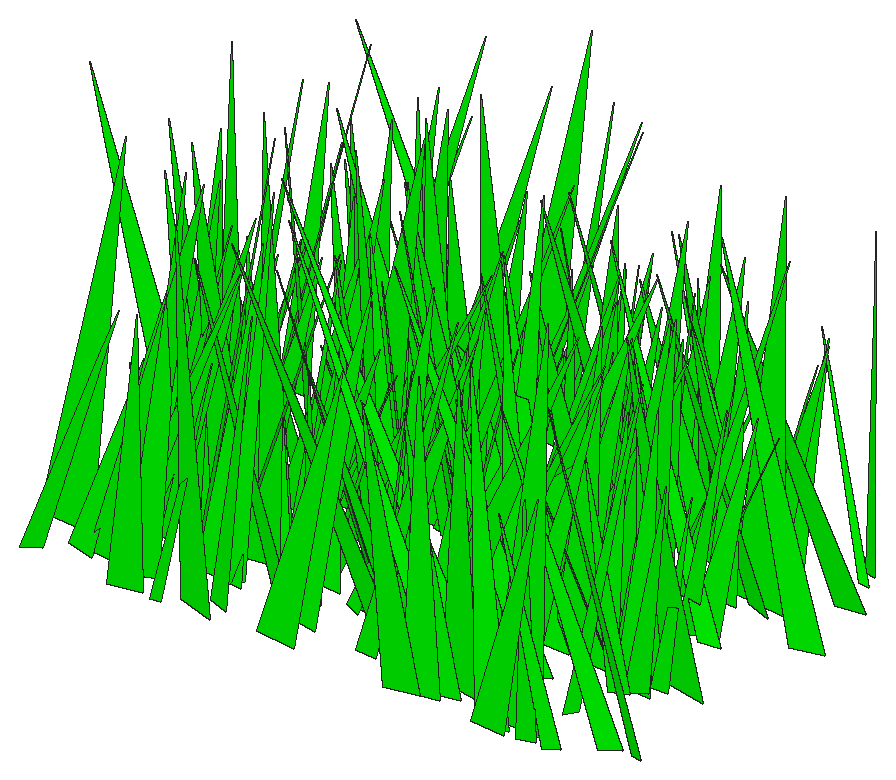
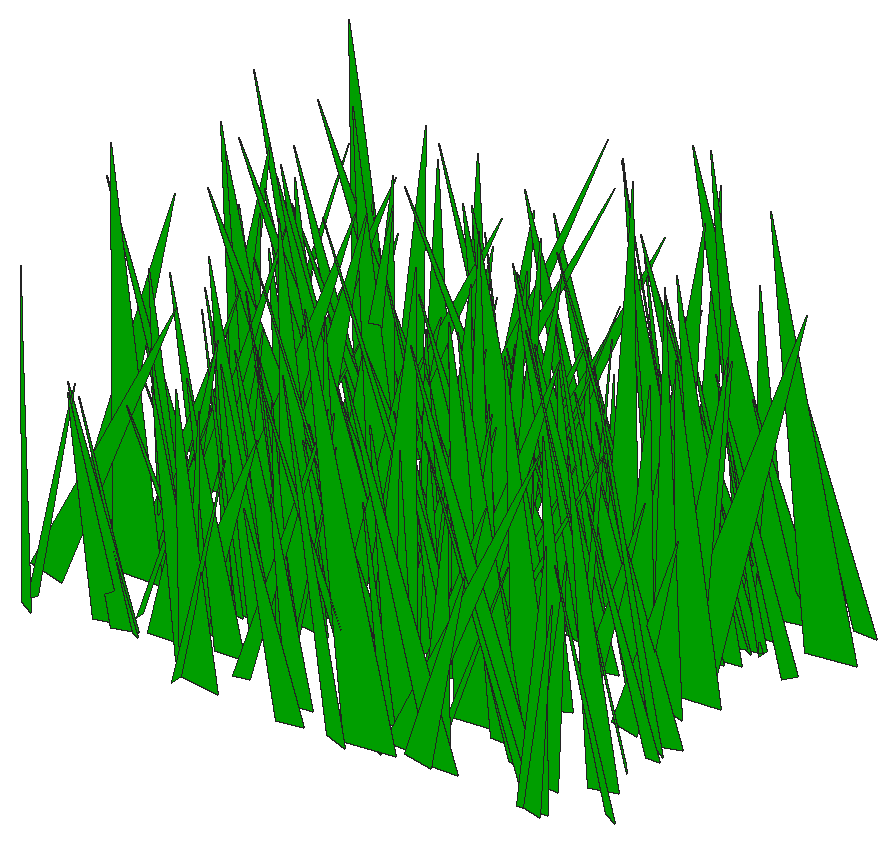
# SketchUp Ruby script. Lengths in inches.
U = 1.inch
M = Sketchup.active_model
def pt(a) = Geom::Point3d.new(a.map { |v| v * U })
def face(e, loops, mat)
  f = e.add_face(loops[0].map { |a| pt(a) })
  loops[1..].each { |l| e.add_face(l.map { |a| pt(a) }).erase! }
  f.material = f.back_material = mat if mat
  f
end
# faces: each face lists its corners as indices into pts; further lists are holes
def faces(e, pts, list, mat = nil) = list.each { |f| face(e, (f[0].is_a?(Array) ? f : [f]).map { |l| l.map { |i| pts[i] } }, mat) }
# xy, xz, yz: faces in a plane at the given z, y or x. An outline is a flat list of corners, or four numbers for a rectangle; further outlines are holes
def ring(l) = l.size == 4 ? [[l[0], l[1]], [l[2], l[1]], [l[2], l[3]], [l[0], l[3]]] : l.each_slice(2).to_a
def flat(e, list, mat, &to3) = list.each { |f| face(e, (f[0].is_a?(Array) ? f : [f]).map { |l| ring(l).map { |u, v| to3.(u, v) } }, mat) }
def xy(e, z, list, mat = nil) = flat(e, list, mat) { |x, y| [x, y, z] }
def xz(e, y, list, mat = nil) = flat(e, list, mat) { |x, z| [x, y, z] }
def yz(e, x, list, mat = nil) = flat(e, list, mat) { |y, z| [x, y, z] }
def lines(e, pts, list) = list.each { |a, b| e.add_line(pt(pts[a]), pt(pts[b])) }
# prism: a flat outline (further loops are holes) pulled along v
def prism(e, loops, v, mat = nil)
  f = face(e, loops, mat); d = Geom::Vector3d.new(v.map { |x| x * U })
  f.pushpull(f.normal.samedirection?(d) ? d.length : -d.length)
end
def box(e, o, s, mat = nil) = prism(e, [[o, [o[0] + s[0], o[1], o[2]], [o[0] + s[0], o[1] + s[1], o[2]], [o[0], o[1] + s[1], o[2]]]], [0, 0, s[2]], mat)
def at(x, y, z, deg = 0) = Geom::Transformation.translation(pt([x, y, z])) * Geom::Transformation.rotation(ORIGIN, Z_AXIS, deg.degrees)
def axes(o, x, y, z) = Geom::Transformation.new([*x, 0, *y, 0, *z, 0, *pt(o).to_a, 1])
def part(name) = M.definitions.add(name)
# library, detail: a bought-in or finely detailed component or shape, given as its bounding box
def library(name, o, s) = part(name).tap { |d| box(d.entities, o, s) }
def detail(e, o, s) = box(e.add_group.entities, o, s)
def put(e, d, t, mat = nil) = e.add_instance(d, t).tap { |i| i.material = mat if mat }
def group(e, t, mat = nil) = e.add_group.tap { |g| g.transformation = t; g.material = mat if mat }.entities
root = M.entities
M.materials.add("[0065_Lime]").color = [0, 255, 0]
c1 = part("fur_instance\#9")
p = [[0.8125,0,1.79],[0.67,-0.02,1.48],[0,-0.11,0],[0,0.11,0]]
faces(c1.entities,p,[[0,1,2,3]])
put(root,c1,axes([128.34,31.92,1.48],[4.60333,0.30174,0.71846],[-2.06784,0.65811,-0.49564],[-1.05614,0.02667,4.10194]),"[0065_Lime]")
put(root,c1,axes([132.14,23.26,1.48],[3.34135,-0.80874,4.77142],[7.14693,0.72519,0.80739],[-4.0565,0.61152,5.35274]),"[0065_Lime]")
put(root,c1,axes([130.33,33.09,1.48],[3.42582,-0.34552,1.24344],[2.23867,0.52713,0.8274],[-1.83612,-0.00196,3.3288]),"[0065_Lime]")
put(root,c1,axes([129.53,30.76,1.48],[4.57043,-0.60507,2.0553],[4.80294,0.66428,-0.51364],[-1.36302,0.31186,5.08182]),"[0065_Lime]")
put(root,c1,axes([130.38,33,1.48],[-1.6277,-0.76836,0.45643],[5.45174,-0.23617,-0.45878],[0.70249,0.05248,4.61797]),"[0065_Lime]")
put(root,c1,axes([131.33,27.52,1.48],[-0.76209,-0.57546,1.29848],[4.33135,-0.05959,0.79707],[-0.74784,0.24132,3.29328]),"[0065_Lime]")
put(root,c1,axes([129.2,20.55,1.48],[2.73963,-1.14979,1.76402],[8.46347,0.36592,-0.70466],[0.16197,0.32736,6.98345]),"[0065_Lime]")
put(root,c1,axes([131.48,24.77,1.48],[2.15394,0.88817,2.66889],[-6.83351,0.39337,-0.73769],[-2.005,-0.38656,5.38135]),"[0065_Lime]")
put(root,c1,axes([129.54,27.59,1.48],[2.27792,-0.51413,0.69377],[3.75514,0.30726,-0.52776],[0.11583,0.1497,3.46584]),"[0065_Lime]")
put(root,c1,axes([130.93,31.66,1.48],[3.10326,-0.47382,1.32397],[3.32885,0.48513,0.65526],[-1.71409,0.08433,3.66951]),"[0065_Lime]")
put(root,c1,axes([129.46,22.14,1.48],[5.53769,-0.24836,1.20733],[2.05402,0.77756,-0.87363],[-1.0526,0.21071,4.64689]),"[0065_Lime]")
put(root,c1,axes([130.65,24.95,1.48],[-0.91208,1.05133,0.76769],[-7.51741,-0.13734,0.3932],[0.59756,-0.12309,6.11825]),"[0065_Lime]")
put(root,c1,axes([129.81,27.9,1.48],[7.16244,0.39874,1.4993],[-2.6458,1.03794,-0.88711],[-2.10942,0.05206,6.2035]),"[0065_Lime]")
put(root,c1,axes([129.52,28.45,1.48],[4.42553,-0.26622,0.25282],[1.84541,0.62013,0.50774],[-0.52949,-0.06376,3.88271]),"[0065_Lime]")
put(root,c1,axes([131.05,25.89,1.48],[6.19126,0.78304,2.67517],[-5.80556,0.95467,-0.47385],[-2.85749,-0.243,6.75895]),"[0065_Lime]")
put(root,c1,axes([129.34,18.78,1.48],[5.67716,-0.44387,0.09403],[3.1183,0.79192,0.69783],[-0.51732,-0.09753,5.23829]),"[0065_Lime]")
put(root,c1,axes([132.54,22.92,1.48],[-4.45383,0.81326,0.35908],[-5.74034,-0.62873,0.60671],[0.86001,0.01513,5.90924]),"[0065_Lime]")
put(root,c1,axes([129.8,29.34,1.48],[8.41541,0.16561,1.42701],[-1.08316,1.207,-0.46748],[-1.81481,0.04755,6.89618]),"[0065_Lime]")
put(root,c1,axes([130.97,21.53,1.48],[4.41636,-0.08561,1.16281],[0.89091,0.63535,-0.67135],[-1.27321,0.14763,3.56366]),"[0065_Lime]")
put(root,c1,axes([130.5625,19.52,1.48],[2.0429,0.57253,0.6611],[-4.14326,0.2713,0.59806],[0.30811,-0.14779,3.6589]),"[0065_Lime]")
put(root,c1,axes([132.06,21.04,1.48],[-2.97248,-0.39475,0.4239],[2.65343,-0.42058,-0.81328],[1.05957,-0.05416,3.22585]),"[0065_Lime]")
put(root,c1,axes([131.73,22.58,1.48],[-0.69959,-1.00839,2.13634],[7.52948,-0.15426,-0.8085],[1.30526,0.34938,5.80895]),"[0065_Lime]")
put(root,c1,axes([131.625,25.6,1.48],[5.15328,0.28882,0.81556],[-1.96634,0.73694,-0.52442],[-1.1677,0.03367,4.4823]),"[0065_Lime]")
put(root,c1,axes([132.04,22.83,1.48],[0.58917,0.85114,0.72485],[-6.09795,0.07036,0.51096],[0.54607,-0.1326,4.92378]),"[0065_Lime]")
put(root,c1,axes([133.82,26.03,1.48],[-2.5746,-0.46803,0.65556],[3.42573,-0.35518,0.40449],[0.08886,0.13248,3.40035]),"[0065_Lime]")
put(root,c1,axes([131.64,21.57,1.48],[6.4084,0.42398,1.01453],[-2.93872,0.91727,-0.56325],[-1.42253,0.01509,5.73396]),"[0065_Lime]")
put(root,c1,axes([131.13,32.37,1.48],[6.37738,0.29659,0.92425],[-2.27645,0.8915,0.80656],[-0.75092,-0.18377,5.40432]),"[0065_Lime]")
put(root,c1,axes([135.83,32.45,1.48],[-6.92423,0.55196,0.38336],[-3.95567,-0.96815,-0.56301],[0.06626,-0.1173,6.45091]),"[0065_Lime]")
put(root,c1,axes([131.21,20.79,1.48],[5.80303,0.48922,0.70277],[-3.57735,0.8063,0.73638],[-0.26469,-0.17187,5.45513]),"[0065_Lime]")
put(root,c1,axes([134.06,26.125,1.48],[-6.81866,-0.24155,2.18598],[2.11875,-1.00909,0.63644],[2.38495,0.20587,5.68441]),"[0065_Lime]")
put(root,c1,axes([132.99,18.57,1.48],[2.80133,-0.81216,0.5112],[5.76495,0.40072,0.4309],[-0.75215,0.04658,5.20662]),"[0065_Lime]")
put(root,c1,axes([133.79,23.86,1.48],[0.88479,0.79255,1.34211],[-5.8248,0.14934,-0.41446],[-0.77866,-0.21659,4.62541]),"[0065_Lime]")
put(root,c1,axes([133.47,27.88,1.48],[-3.77573,0.57189,1.48796],[-4.02313,-0.58196,0.74051],[1.92998,-0.09429,4.45461]),"[0065_Lime]")
put(root,c1,axes([131.58,21.66,1.48],[5.32402,-0.84632,0.62711],[6.07161,0.74374,-0.47181],[-0.07269,0.13519,6.52173]),"[0065_Lime]")
put(root,c1,axes([131.82,19.61,1.48],[3.4087,-1.22529,0.85308],[8.76381,0.46417,-0.829],[0.57558,0.18891,7.57027]),"[0065_Lime]")
put(root,c1,axes([134.16,22.28,1.48],[-2.68174,-0.47401,0.38631],[3.32939,-0.38268,-0.44206],[0.72118,0.00401,3.47735]),"[0065_Lime]")
put(root,c1,axes([134.42,22.16,1.48],[0.56166,-1.21816,1.28586],[8.75698,0.102,0.70717],[-0.9835,0.21253,7.03085]),"[0065_Lime]")
put(root,c1,axes([132,31.34,1.48],[6.54368,0.88682,0.28379],[-6.24469,0.91797,-0.85246],[-0.97751,0.07227,7.34559]),"[0065_Lime]")
put(root,c1,axes([132.52,25.26,1.48],[3.161,-0.6405,1.13017],[4.76521,0.42484,-0.75046],[0.00081,0.23436,4.44911]),"[0065_Lime]")
put(root,c1,axes([134.83,32.79,1.48],[-0.68585,0.6153,0.77968],[-4.41654,-0.06947,-0.73334],[-0.76607,-0.15034,3.52983]),"[0065_Lime]")
put(root,c1,axes([135.2,31.17,1.48],[-4.35569,0.1387,0.30321],[-0.92484,-0.60898,0.54454],[0.50791,0.08062,3.59177]),"[0065_Lime]")
put(root,c1,axes([132.93,19.45,1.48],[7.34664,-0.69558,1.83397],[4.95791,1.07532,0.52563],[-2.23744,0.09886,7.18659]),"[0065_Lime]")
put(root,c1,axes([133.46,29.125,1.48],[-1.67518,-0.97817,1.81289],[7.15511,-0.28509,-0.78004],[1.49324,0.26872,5.77148]),"[0065_Lime]")
put(root,c1,axes([134.37,32.62,1.48],[2.47895,-0.72311,0.28405],[5.03355,0.35104,0.88023],[-1.12555,-0.02271,4.56206]),"[0065_Lime]")
put(root,c1,axes([136.79,27.39,1.48],[-6.12157,0.04266,0.22323],[-0.34433,-0.84935,-0.80808],[0.22121,-0.14145,4.91956]),"[0065_Lime]")
put(root,c1,axes([133.38,30.36,1.48],[6.16272,-0.7472,1.14624],[5.29014,0.88653,0.54645],[-1.50867,0.05638,6.59836]),"[0065_Lime]")
put(root,c1,axes([133.48,21.38,1.48],[8.89591,0.24035,1.99762],[-1.54398,1.29568,-0.67455],[-2.56378,0.05368,7.33765]),"[0065_Lime]")
put(root,c1,axes([134.12,18.58,1.48],[4.80932,0.35635,0.69921],[-2.41076,0.6843,-0.71499],[-1.16545,0.05502,4.36432]),"[0065_Lime]")
put(root,c1,axes([135.37,18.89,1.48],[5.33626,0.61922,3.60877],[-5.67244,0.82426,0.81046],[-2.63166,-0.52106,5.57065]),"[0065_Lime]")
put(root,c1,axes([136.58,30.45,1.48],[-2.65795,0.65882,0.18406],[-4.68262,-0.36961,-0.40861],[-0.32628,-0.06238,4.36482]),"[0065_Lime]")
put(root,c1,axes([135.65,22.32,1.48],[5.64928,0.92654,2.8004],[-6.8319,0.88657,-0.71033],[-2.94199,-0.27963,7.02693]),"[0065_Lime]")
put(root,c1,axes([134.76,20.74,1.48],[-0.67276,1.03413,0.78932],[-7.36111,-0.1106,0.70424],[0.95733,-0.12368,5.9698]),"[0065_Lime]")
put(root,c1,axes([133.99,25.3,1.48],[2.82182,-0.79631,0.87958],[5.76412,0.382,-0.64637],[0.24345,0.18544,5.10874]),"[0065_Lime]")
put(root,c1,axes([137.02,20.875,1.48],[-5.77141,-0.41097,1.13216],[3.14285,-0.80719,0.78195],[0.78328,0.21068,5.2045]),"[0065_Lime]")
put(root,c1,axes([137.66,27.66,1.48],[-5.41557,0.82192,0.41597],[-5.8715,-0.75793,-0.39443],[-0.00976,-0.09902,6.47194]),"[0065_Lime]")
put(root,c1,axes([134.79,30,1.48],[1.22293,-1.15319,0.59658],[8.23032,0.16607,-0.40623],[0.38799,0.11213,6.73695]),"[0065_Lime]")
put(root,c1,axes([135.93,28.42,1.48],[1.141,0.84619,1.29458],[-6.17553,0.18334,-0.41433],[-0.81233,-0.2052,4.96825]),"[0065_Lime]")
put(root,c1,axes([133.9,32.74,1.48],[5.46387,0.74694,1.24285],[-5.50814,0.76219,0.6723],[-0.50091,-0.23374,6.16407]),"[0065_Lime]")
put(root,c1,axes([134.24,32.21,1.48],[5.25032,-0.14543,0.54963],[0.97645,0.74207,0.4078],[-0.75777,-0.05138,4.33371]),"[0065_Lime]")
put(root,c1,axes([135.15,23.66,1.48],[6.02917,-0.06436,1.52648],[0.7062,0.87787,-0.60529],[-1.798,0.12899,4.88094]),"[0065_Lime]")
put(root,c1,axes([134.24,22.12,1.48],[7.25404,0.04386,0.9317],[-0.21361,1.0285,-0.52188],[-1.16781,0.08429,5.88289]),"[0065_Lime]")
put(root,c1,axes([135.27,20.78,1.48],[7.95708,-0.43814,1.8997],[2.92689,1.16489,0.89124],[-2.57094,-0.02986,6.89421]),"[0065_Lime]")
put(root,c1,axes([137.4,28.45,1.48],[-5.51712,0.44821,0.73572],[-3.0677,-0.7837,0.7778],[1.25757,0.0546,5.12505]),"[0065_Lime]")
put(root,c1,axes([135.32,24.37,1.48],[4.68672,0.94892,0.53479],[-6.71887,0.66472,-0.56357],[-0.94454,-0.01994,6.66246]),"[0065_Lime]")
put(root,c1,axes([135.77,19.45,1.48],[5.293,0.39714,1.79325],[-3.16704,0.77689,0.41967],[-1.67863,-0.21351,4.86264]),"[0065_Lime]")
put(root,c1,axes([135.51,27.42,1.48],[2.61079,-0.54396,0.68352],[3.96071,0.36085,-0.38662],[-0.06703,0.13533,3.77829]),"[0065_Lime]")
put(root,c1,axes([138.29,24.8,1.48],[-3.82193,-0.22686,0.29797],[1.65362,-0.52934,0.52871],[0.07937,0.10425,3.33314]),"[0065_Lime]")
put(root,c1,axes([137.02,27.23,1.48],[-7.05338,0.49513,3.51961],[-4.46681,-1.08833,-0.79247],[3.34453,-0.40934,6.36423]),"[0065_Lime]")
put(root,c1,axes([135.71,26.32,1.48],[2.63387,-1.2713,0.40545],[9.04927,0.36535,-0.50768],[0.46108,0.09165,7.64787]),"[0065_Lime]")
put(root,c1,axes([136.49,31.3125,1.48],[1.55089,-0.76196,1.56092],[5.75138,0.20102,-0.49267],[0.09049,0.28248,4.5611]),"[0065_Lime]")
put(root,c1,axes([137.81,24.625,1.48],[-6.16782,-0.64416,2.56529],[5.11849,-0.91629,0.43255],[2.18222,0.32855,6.23598]),"[0065_Lime]")
put(root,c1,axes([135.99,28.99,1.48],[4.50663,0.44035,0.9326],[-3.29555,0.62983,0.57168],[-0.52367,-0.17405,4.42815]),"[0065_Lime]")
put(root,c1,axes([137.71,24.16,1.48],[3.78951,0.28839,1.48428],[-1.86774,0.59099,-0.69263],[-2.01328,-0.00545,3.43635]),"[0065_Lime]")
put(root,c1,axes([136.37,33.11,1.48],[0.03356,-1.06692,3.84207],[8.86127,-0.08506,-0.84271],[1.19943,0.65826,6.11837]),"[0065_Lime]")
put(root,c1,axes([138.09,27.19,1.48],[1.40454,1.14815,1.28321],[-8.21685,0.22693,-0.85313],[-1.31732,-0.1913,6.6896]),"[0065_Lime]")
put(root,c1,axes([136.92,31.55,1.48],[4.01358,-0.25979,0.64462],[1.66637,0.56863,0.81429],[-1.12659,-0.08443,3.50095]),"[0065_Lime]")
put(root,c1,axes([137.54,22.27,1.48],[-2.13721,0.63206,0.75339],[-4.46718,-0.31942,0.59503],[1.06525,-0.07141,4.00684]),"[0065_Lime]")
put(root,c1,axes([137.9,20.03,1.48],[-3.32331,0.33092,0.8524],[-2.2362,-0.48964,0.60117],[1.28205,0.00377,3.25815]),"[0065_Lime]")
put(root,c1,axes([137.6,21.5,1.48],[-2.98356,-0.5352,0.94271],[3.69535,-0.44801,-0.78477],[1.48132,0.03966,3.85643]),"[0065_Lime]")
put(root,c1,axes([138.65,26.9,1.48],[-0.73993,-0.67483,1.00542],[4.91022,-0.07513,0.70109],[-0.69375,0.18797,3.88982]),"[0065_Lime]")
put(root,c1,axes([136.25,23.04,1.48],[4.71944,0.20483,0.37539],[-1.50184,0.66048,0.41651],[-0.2868,-0.08808,3.99614]),"[0065_Lime]")
put(root,c1,axes([140.02,21.9,1.48],[-6.55893,-0.14654,0.67817],[1.16059,-0.9161,0.79354],[0.66006,0.15464,5.34354]),"[0065_Lime]")
put(root,c1,axes([138.23,29.17,1.48],[3.98517,-0.22604,1.99179],[2.2839,0.60353,-0.72834],[-1.83509,0.26025,3.419]),"[0065_Lime]")
put(root,c1,axes([139.46,27.05,1.48],[-3.06982,-0.78935,1.54631],[5.93036,-0.40815,0.80812],[-0.00886,0.3014,5.14397]),"[0065_Lime]")
put(root,c1,axes([137.67,27.94,1.48],[0.54886,0.6103,1.20616],[-4.56971,0.05327,0.47268],[0.42443,-0.2157,3.52942]),"[0065_Lime]")
put(root,c1,axes([138.57,29.33,1.48],[2.23122,-1.1329,1.94492],[8.30358,0.35178,0.56363],[-1.33011,0.29569,6.78114]),"[0065_Lime]")
put(root,c1,axes([137.43,33.35,1.48],[6.22868,0.52704,1.48257],[-3.72886,0.91002,-0.47506],[-1.86697,-0.05921,5.89505]),"[0065_Lime]")
put(root,c1,axes([136.41,32.92,1.48],[6.92028,0.50093,0.43633],[-3.48192,0.97103,-0.8172],[-0.93404,0.09157,6.27908]),"[0065_Lime]")
put(root,c1,axes([141.18,20.66,1.48],[-6.0567,-0.73133,0.15907],[5.19671,-0.84579,0.61648],[-0.34645,0.09863,6.46635]),"[0065_Lime]")
put(root,c1,axes([139.13,24.375,1.48],[-5.61723,0.00055,1.46852],[0.25505,-0.82053,0.65573],[1.78728,0.11881,4.52183]),"[0065_Lime]")
put(root,c1,axes([139.39,22.71,1.48],[3.93737,0.62008,2.90977],[-4.94259,0.67542,-0.39796],[-2.80008,-0.32029,4.79408]),"[0065_Lime]")
put(root,c1,axes([137.1875,22.76,1.48],[4.87272,-0.13442,0.49945],[0.84498,0.68237,0.69955],[-0.76035,-0.10312,3.97815]),"[0065_Lime]")
put(root,c1,axes([139.19,23.51,1.48],[-5.59938,0.56591,1.57879],[-4.06445,-0.82644,0.38887],[1.86191,-0.10221,5.59683]),"[0065_Lime]")
put(root,c1,axes([136.91,21.67,1.48],[2.85352,-0.77982,0.47223],[5.54528,0.38613,-0.80372],[0.6204,0.1354,5.01186]),"[0065_Lime]")
put(root,c1,axes([138.46,27.58,1.48],[-0.86545,-0.58758,0.30401],[4.14903,-0.12789,-0.4682],[0.64086,0.0345,3.44172]),"[0065_Lime]")
put(root,c1,axes([140.29,25.29,1.48],[-6.67867,-0.2442,1.58221],[2.04353,-0.95677,0.75908],[1.62102,0.20005,5.56186]),"[0065_Lime]")
put(root,c1,axes([138.01,20.18,1.48],[1.53713,1.01323,1.34733],[-7.35825,0.1846,0.90247],[0.77075,-0.25836,5.92878]),"[0065_Lime]")
put(root,c1,axes([141.24,21.3125,1.48],[-3.63239,-0.54543,0.26173],[3.88825,-0.50419,0.49577],[-0.22743,0.09142,4.29567]),"[0065_Lime]")
put(root,c1,axes([138.32,18.93,1.48],[2.47007,-0.79715,1.37659],[5.90874,0.3161,-0.88124],[0.36462,0.27767,4.95512]),"[0065_Lime]")
put(root,c1,axes([139.12,33.41,1.48],[-0.07266,0.68458,0.01899],[-4.81532,-0.01059,0.60184],[0.74017,-0.00169,3.91728]),"[0065_Lime]")
put(root,c1,axes([138.87,29.28,1.48],[0.85824,0.58263,0.32577],[-4.10574,0.10861,0.64769],[0.70348,-0.07691,3.38268]),"[0065_Lime]")
put(root,c1,axes([140.83,31.33,1.48],[-5.12571,-0.12843,1.15635],[1.11108,-0.73676,0.51659],[1.27351,0.12588,4.20346]),"[0065_Lime]")
put(root,c1,axes([139.52,32.43,1.48],[-0.09125,0.63537,0.53923],[-4.5427,-0.02278,0.39085],[0.49884,-0.09123,3.65791]),"[0065_Lime]")
put(root,c1,axes([143.59,21.29,1.48],[-8.7011,0.45759,0.13498],[-3.26057,-1.22055,-0.41578],[-0.02401,-0.07544,7.54557]),"[0065_Lime]")
put(root,c1,axes([136.97,23.14,1.48],[7.6362,-0.40029,0.27915],[2.86917,1.0666,-0.67903],[-0.02781,0.12677,6.59466]),"[0065_Lime]")
put(root,c1,axes([137.61,30.51,1.48],[8.56832,0.14589,0.85467],[-0.96055,1.21053,-0.55245],[-1.12216,0.07774,6.99879]),"[0065_Lime]")
put(root,c1,axes([138.79,23.68,1.48],[4.02392,0.6007,0.87584],[-4.40813,0.55073,0.74284],[-0.05294,-0.19825,4.7173]),"[0065_Lime]")
put(root,c1,axes([138.11,26.93,1.48],[7.82637,0.49209,0.68157],[-3.46549,1.10586,-0.42508],[-0.97787,0.01935,6.96135]),"[0065_Lime]")
put(root,c1,axes([141.96,32.12,1.48],[-5.48275,-0.49958,0.3642],[3.46044,-0.76803,-0.83465],[0.9306,-0.08746,5.24938]),"[0065_Lime]")
put(root,c1,axes([138.9375,21.76,1.48],[4.43931,0.30928,0.45627],[-2.26767,0.61338,0.66583],[-0.12972,-0.13824,3.97508]),"[0065_Lime]")
put(root,c1,axes([140.03,21.77,1.48],[0.43339,1.00053,1.51648],[-7.32332,0.03233,0.66995],[0.73721,-0.26701,5.76366]),"[0065_Lime]")
put(root,c1,axes([141.9,20.92,1.48],[-1.58505,-0.5723,0.74779],[4.16197,-0.20556,0.56539],[-0.33275,0.15505,3.50965]),"[0065_Lime]")
put(root,c1,axes([140.2,28.89,1.48],[2.93314,0.42551,1.18243],[-3.34714,0.39304,0.75402],[-0.28232,-0.23899,3.34529]),"[0065_Lime]")
put(root,c1,axes([140.32,29.09,1.48],[0.5523,-0.57643,0.59622],[4.08079,0.05377,-0.75919],[0.8441,0.11722,3.28018]),"[0065_Lime]")
put(root,c1,axes([144.34,19.48,1.48],[-8.70337,0.36697,0.66462],[-2.67212,-1.22225,-0.53792],[0.5897,-0.12228,7.37168]),"[0065_Lime]")
put(root,c1,axes([140.83,23.52,1.48],[-1.56201,0.55497,1.21751],[-4.01823,-0.26434,0.62676],[1.30107,-0.15012,3.39737]),"[0065_Lime]")
put(root,c1,axes([140.82,20.5625,1.48],[5.72571,0.12092,1.57988],[-1.1088,0.83935,0.50601],[-1.81208,-0.13151,4.68241]),"[0065_Lime]")
put(root,c1,axes([142.71,25.79,1.48],[-5.17594,-0.43241,1.53984],[3.455,-0.7283,0.83082],[1.05647,0.26329,4.82708]),"[0065_Lime]")
put(root,c1,axes([141.5,23.89,1.48],[3.68649,-0.44695,1.13642],[3.14384,0.55101,0.51391],[-1.47823,0.05723,3.92703]),"[0065_Lime]")
put(root,c1,axes([141.48,30.61,1.48],[-4.1994,0.38125,1.73097],[-2.71098,-0.65623,0.49165],[2.1308,-0.08355,4.03692]),"[0065_Lime]")
put(root,c1,axes([141.89,20.35,1.48],[2.41586,0.55675,0.73888],[-3.90003,0.35933,-0.6356],[-1.14596,-0.04918,3.72079]),"[0065_Lime]")
put(root,c1,axes([140.37,24.16,1.48],[3.18981,0.5414,0.22314],[-3.84114,0.43934,0.61154],[0.40702,-0.09683,4.02244]),"[0065_Lime]")
put(root,c1,axes([142.65,28.3,1.48],[2.16656,-0.5513,0.83341],[3.79661,0.33313,0.85394],[-1.42424,0.04937,3.54416]),"[0065_Lime]")
put(root,c1,axes([143.36,33.4,1.48],[-5.16194,0.14461,0.82736],[-0.83667,-0.73034,0.82361],[1.18052,0.11469,4.20145]),"[0065_Lime]")
put(root,c1,axes([142.44,27.35,1.48],[4.17393,0.61671,1.51786],[-4.36224,0.63453,-0.70217],[-1.92738,-0.10059,4.8763]),"[0065_Lime]")
put(root,c1,axes([140.9375,19.88,1.48],[6.48036,0.60279,0.85205],[-4.24188,0.92241,-0.52084],[-1.22713,-0.00527,6.3]),"[0065_Lime]")
put(root,c1,axes([141.95,29.66,1.48],[5.6458,0.01589,1.53706],[0.118,0.83067,-0.5746],[-1.88934,0.09937,4.55721]),"[0065_Lime]")
put(root,c1,axes([143.1,18.83,1.48],[0.81302,-0.87911,0.4167],[6.21391,0.123,0.6734],[-0.88911,0.05573,5.08734]),"[0065_Lime]")
put(root,c1,axes([141.39,22.96,1.48],[6.17368,0.02961,1.1127],[0.01685,0.87701,-0.84377],[-1.38397,0.14274,4.95333]),"[0065_Lime]")
put(root,c1,axes([142.65,33.23,1.48],[1.58731,0.95071,0.07014],[-6.74089,0.22327,-0.47322],[-0.58607,0.00692,5.63295]),"[0065_Lime]")
put(root,c1,axes([145.71,21.96,1.48],[-6.55572,0.61074,0.3084],[-4.36081,-0.91432,-0.65905],[-0.13391,-0.12428,6.36398]),"[0065_Lime]")
put(root,c1,axes([142.4,28.62,1.48],[4.09581,-1.06576,0.22427],[7.53337,0.57624,0.73108],[-0.92154,-0.02614,6.97322]),"[0065_Lime]")
put(root,c1,axes([144.6875,31.16,1.48],[-1.74093,0.68995,0.34294],[-4.86353,-0.2304,-0.8033],[-0.7955,-0.10135,4.16071]),"[0065_Lime]")
put(root,c1,axes([142.46,27.72,1.48],[4.58822,-0.3355,0.66419],[2.26116,0.65233,0.70676],[-1.12011,-0.05743,4.14742]),"[0065_Lime]")
put(root,c1,axes([144.27,19.36,1.48],[-0.75524,0.76394,1.0295],[-5.54691,-0.08263,-0.6378],[-0.62467,-0.18991,4.41887]),"[0065_Lime]")
put(root,c1,axes([144.72,22.01,1.48],[-1.17695,0.74008,0.03525],[-5.19144,-0.16195,-0.74846],[-0.88871,-0.03405,4.32545]),"[0065_Lime]")
put(root,c1,axes([142.54,29.35,1.48],[-1.78934,-0.67037,1.86729],[4.93761,-0.33417,-0.88948],[1.91038,0.23581,4.04795]),"[0065_Lime]")
put(root,c1,axes([142.92,23.97,1.48],[-6.1574,0.7622,3.42774],[-5.87446,-0.99647,0.44282],[3.55963,-0.32603,6.66003]),"[0065_Lime]")
put(root,c1,axes([142.81,29.98,1.48],[3.17966,-0.58099,1.33543],[4.41872,0.4453,-0.46933],[-0.51519,0.23357,4.21662]),"[0065_Lime]")
put(root,c1,axes([142.74,28.6875,1.48],[6.15785,0.18671,1.59091],[-1.63066,0.89053,0.67403],[-1.71223,-0.17664,5.07962]),"[0065_Lime]")
put(root,c1,axes([143.04,31.3,1.48],[1.52719,0.72174,1.29745],[-5.37682,0.19954,0.46808],[0.12354,-0.23764,4.33347]),"[0065_Lime]")
put(root,c1,axes([144.92,23.59,1.48],[-5.86835,0.72885,0.88738],[-5.11234,-0.8387,0.7141],[1.39927,-0.00756,6.33056]),"[0065_Lime]")
put(root,c1,axes([143.72,18.98,1.48],[3.07864,-0.84131,1.39266],[6.09479,0.46214,0.4405],[-1.27734,0.17736,5.45844]),"[0065_Lime]")
put(root,c1,axes([144.09,31.79,1.48],[-4.21242,-0.28926,1.78892],[2.50119,-0.63194,0.47276],[1.67884,0.21569,3.78428]),"[0065_Lime]")
put(root,c1,axes([143.51,32.46,1.48],[0.57019,0.77562,1.18092],[-5.68856,0.06057,0.48429],[0.46385,-0.21064,4.48764]),"[0065_Lime]")
put(root,c1,axes([142.47,25.34,1.48],[5.565,-0.7572,1.27439],[5.59335,0.77352,-0.75988],[-0.4543,0.24824,6.25503]),"[0065_Lime]")
put(root,c1,axes([145.01,22.08,1.48],[-4.12555,0.9134,0.99392],[-6.49916,-0.5974,0.54761],[1.22779,-0.09309,6.23843]),"[0065_Lime]")
put(root,c1,axes([146.62,26.74,1.48],[-5.38749,-0.91517,0.73555],[6.57513,-0.75118,0.54578],[0.0546,0.15804,6.85358]),"[0065_Lime]")
put(root,c1,axes([145.25,31.68,1.48],[-3.94018,-0.78933,0.29951],[5.54936,-0.55524,-0.73018],[0.9456,-0.03054,5.53319]),"[0065_Lime]")
put(root,c1,axes([143.8,29.16,1.48],[0.81502,1.01286,1.53344],[-7.43759,0.0949,0.51501],[0.43904,-0.27255,5.878]),"[0065_Lime]")
put(root,c1,axes([144.42,19.92,1.48],[-2.35853,-0.90746,0.99293],[6.44546,-0.355,-0.74186],[1.28515,0.11504,5.54294]),"[0065_Lime]")
put(root,c1,axes([142.28,23.37,1.48],[6.60797,-0.23809,0.46282],[1.75524,0.92219,-0.68461],[-0.33718,0.13467,5.5065]),"[0065_Lime]")
put(root,c1,axes([145.96,24.95,1.48],[-1.27273,-1.03767,1.03165],[7.44337,-0.15438,0.87249],[-0.85889,0.19978,6.03255]),"[0065_Lime]")
put(root,c1,axes([143.16,24.94,1.48],[2.57471,-1.0903,0.17125],[7.71129,0.35574,-0.81527],[0.88579,0.07224,6.59963]),"[0065_Lime]")
put(root,c1,axes([144.25,29.32,1.48],[5.63629,0.19326,1.57641],[-1.65785,0.82197,0.54523],[-1.70264,-0.1606,4.68755]),"[0065_Lime]")
put(root,c1,axes([142.2,21.62,1.48],[6.56789,-0.74744,0.20516],[5.32219,0.91947,-0.48302],[0.17838,0.08712,6.85772]),"[0065_Lime]")
put(root,c1,axes([146.58,31.08,1.48],[-5.1509,0.06964,0.59054],[-0.427,-0.7283,0.41371],[0.76835,0.06211,4.18878]),"[0065_Lime]")
put(root,c1,axes([142.58,24.35,1.48],[5.42595,0.94508,0.38993],[-6.72566,0.75243,0.81269],[0.47983,-0.14036,6.98199]),"[0065_Lime]")
put(root,c1,axes([144.86,24.84,1.48],[-1.64535,-0.60668,1.1841],[4.39465,-0.26872,-0.57325],[1.20279,0.15193,3.71428]),"[0065_Lime]")
put(root,c1,axes([144.74,28.68,1.48],[0.34114,-0.75623,0.94754],[5.48004,0.03061,-0.48679],[0.53779,0.16779,4.35927]),"[0065_Lime]")
put(root,c1,axes([144.99,21.86,1.48],[4.77084,-0.5563,0.91978],[3.83297,0.6889,0.8076],[-1.50343,-0.00897,4.9777]),"[0065_Lime]")
put(root,c1,axes([144.23,30.7,1.48],[4.44699,-0.05888,0.35609],[0.49278,0.61652,-0.65572],[-0.35269,0.11899,3.5736]),"[0065_Lime]")
put(root,c1,axes([146.47,26.97,1.48],[-4.40774,0.44303,0.79039],[-3.08638,-0.63422,0.52441],[1.16577,-0.00402,4.37682]),"[0065_Lime]")
put(root,c1,axes([146.45,18.88,1.48],[-5.07535,0.71221,1.46769],[-5.10522,-0.74753,0.47463],[1.69767,-0.11874,5.8151]),"[0065_Lime]")
put(root,c1,axes([144.86,24.3125,1.48],[2.68944,-0.85842,1.66612],[6.43998,0.34817,-0.86695],[0.20565,0.32317,5.35972]),"[0065_Lime]")
put(root,c1,axes([145.5,30.35,1.48],[2.95604,0.54159,1.81311],[-4.41389,0.40579,0.69964],[-0.58415,-0.32554,3.88855]),"[0065_Lime]")
put(root,c1,axes([145.64,23.6875,1.48],[-0.03291,-0.91091,2.36753],[7.07865,-0.04003,-0.45093],[0.62239,0.40705,5.25371]),"[0065_Lime]")
put(root,c1,axes([147.86,23,1.48],[-4.23021,-0.15304,0.07732],[1.07014,-0.59056,-0.43153],[0.22368,-0.0689,3.52682]),"[0065_Lime]")
put(root,c1,axes([148.4,26.58,1.48],[-7.2041,0.42751,0.70718],[-2.99096,-1.01919,0.4862],[1.03254,0.03046,6.34243]),"[0065_Lime]")
put(root,c1,axes([143.92,25.11,1.48],[5.00614,-0.74582,0.11222],[5.26941,0.69464,-0.83258],[0.65102,0.11267,5.87604]),"[0065_Lime]")
put(root,c1,axes([148.26,29.04,1.48],[-5.65203,-0.56702,0.29889],[3.99126,-0.79437,-0.56046],[0.6985,-0.04905,5.62101]),"[0065_Lime]")
put(root,c1,axes([146.08,24.21,1.48],[0.25105,-0.58023,0.06376],[4.09449,0.03352,-0.4439],[0.5401,0.01555,3.33555]),"[0065_Lime]")
put(root,c1,axes([145.41,21.33,1.48],[4.16168,0.79096,0.97062],[-5.74883,0.5803,0.46277],[-0.24298,-0.18259,5.67527]),"[0065_Lime]")
put(root,c1,axes([145.95,32.07,1.48],[4.59637,-0.09075,0.53505],[0.49246,0.63908,0.83317],[-0.77927,-0.13141,3.6824]),"[0065_Lime]")
put(root,c1,axes([146.8,23.49,1.48],[-0.17179,0.75979,1.04738],[-5.53328,-0.04052,0.38454],[0.52644,-0.17798,4.38356]),"[0065_Lime]")
put(root,c1,axes([146.11,25.26,1.48],[2.21509,-1.08258,0.29675],[7.70296,0.30781,-0.41523],[0.39051,0.06901,6.50735]),"[0065_Lime]")
put(root,c1,axes([146.375,32.01,1.48],[0.27901,0.62937,1.51919],[-4.73947,-0.02112,0.86906],[1.04223,-0.26451,3.5453]),"[0065_Lime]")
put(root,c1,axes([147.03,28.84,1.48],[4.26013,-0.55816,2.23156],[4.60387,0.62442,-0.58164],[-1.45233,0.34214,4.70205]),"[0065_Lime]")
put(root,c1,axes([148.14,22.7,1.48],[-3.37035,0.40855,1.50448],[-3.33388,-0.47855,-0.58691],[0.87159,-0.25066,3.57274]),"[0065_Lime]")
put(root,c1,axes([146.43,18.67,1.48],[1.62107,-0.76546,0.49713],[5.45667,0.2168,-0.58688],[0.52261,0.11073,4.58567]),"[0065_Lime]")
put(root,c1,axes([147.09,31.95,1.48],[-1.10205,0.70535,0.25767],[-4.91435,-0.16071,0.83457],[1.07061,-0.01163,4.09612]),"[0065_Lime]")
put(root,c1,axes([147.79,18.8,1.48],[-3.67015,-0.40618,2.38205],[3.84848,-0.53399,0.8721],[1.45625,0.3875,3.69867]),"[0065_Lime]")
put(root,c1,axes([147.08,19.22,1.48],[1.43212,-1.14178,2.49038],[8.68297,0.18494,-0.46248],[0.06709,0.43747,6.69535]),"[0065_Lime]")
put(root,c1,axes([148.68,18.86,1.48],[-3.67933,0.3515,1.12216],[-2.78912,-0.51036,-0.69377],[0.61765,-0.21074,3.55187]),"[0065_Lime]")
put(root,c1,axes([145.92,28.39,1.48],[7.72553,-0.22817,1.29007],[1.84649,1.09155,-0.84687],[-1.3201,0.19147,6.36527]),"[0065_Lime]")
put(root,c1,axes([150.05,19.89,1.48],[-5.47605,0.5022,0.72006],[-3.67807,-0.7563,-0.83229],[0.16786,-0.18865,5.25347]),"[0065_Lime]")
put(root,c1,axes([150.3125,30.77,1.48],[-4.01844,-0.79734,0.20203],[5.63914,-0.55499,0.8168],[-0.67797,0.10978,5.59646]),"[0065_Lime]")
put(root,c1,axes([148.36,24,1.48],[3.24291,-0.68,1.61171],[4.94383,0.50544,0.56421],[-1.70382,0.17234,4.70472]),"[0065_Lime]")
put(root,c1,axes([147.28,24.66,1.48],[4.10103,-1.01728,0.37879],[7.21833,0.57971,0.46172],[-0.72366,0.01743,6.75218]),"[0065_Lime]")
put(root,c1,axes([147.49,26.63,1.48],[4.61035,-0.42421,0.52836],[2.90895,0.65166,0.73763],[-1.03623,-0.05802,4.42147]),"[0065_Lime]")
put(root,c1,axes([148.04,29.36,1.48],[-1.24534,-1.13965,2.68619],[8.67835,-0.22326,-0.51191],[1.17027,0.44285,6.65471]),"[0065_Lime]")
put(root,c1,axes([148.34,23.06,1.48],[-0.97731,0.80649,1.29122],[-5.89393,-0.16327,0.46562],[0.85008,-0.20483,4.71279]),"[0065_Lime]")
put(root,c1,axes([149.69,32.16,1.48],[-4.83951,0.18741,0.83647],[-1.17595,-0.69077,0.68453],[1.20559,0.07852,4.02549]),"[0065_Lime]")
put(root,c1,axes([147.3125,27.01,1.48],[4.79578,0.16077,0.22606],[-1.07959,0.66581,-0.71328],[-0.46984,0.11113,3.94648]),"[0065_Lime]")
put(root,c1,axes([148,26.79,1.48],[-0.48652,0.71983,0.5048],[-5.02862,-0.08579,0.8925],[1.15756,-0.07013,4.08934]),"[0065_Lime]")
put(root,c1,axes([149.58,23.9,1.48],[-3.78576,-0.97421,0.31129],[6.88638,-0.53463,-0.65443],[0.88942,-0.00729,6.39197]),"[0065_Lime]")
put(root,c1,axes([150.88,28.05,1.48],[-5.92297,0.73869,1.2938],[-5.43196,-0.83645,-0.45053],[0.81169,-0.20737,6.42596]),"[0065_Lime]")
put(root,c1,axes([147.78,20.89,1.48],[7.39795,-0.29338,1.2764],[1.96929,1.06165,0.62499],[-1.71564,-0.04646,6.22133]),"[0065_Lime]")
put(root,c1,axes([150.94,20,1.48],[-6.36233,-0.28953,1.05731],[2.20877,-0.90104,0.52602],[1.02784,0.14408,5.41433]),"[0065_Lime]")
put(root,c1,axes([148.52,23.01,1.48],[3.78667,-0.54621,0.02646],[3.8019,0.52172,0.89486],[-0.81027,-0.10467,4.32247]),"[0065_Lime]")
put(root,c1,axes([148.96,23.54,1.48],[2.88855,0.44877,0.49203],[-3.15319,0.41448,-0.41986],[-0.78941,-0.01345,3.47749]),"[0065_Lime]")
put(root,c1,axes([149.47,32.75,1.48],[-6.17998,-0.25796,2.58777],[2.31084,-0.95317,0.46749],[2.85503,0.21312,5.22309]),"[0065_Lime]")
